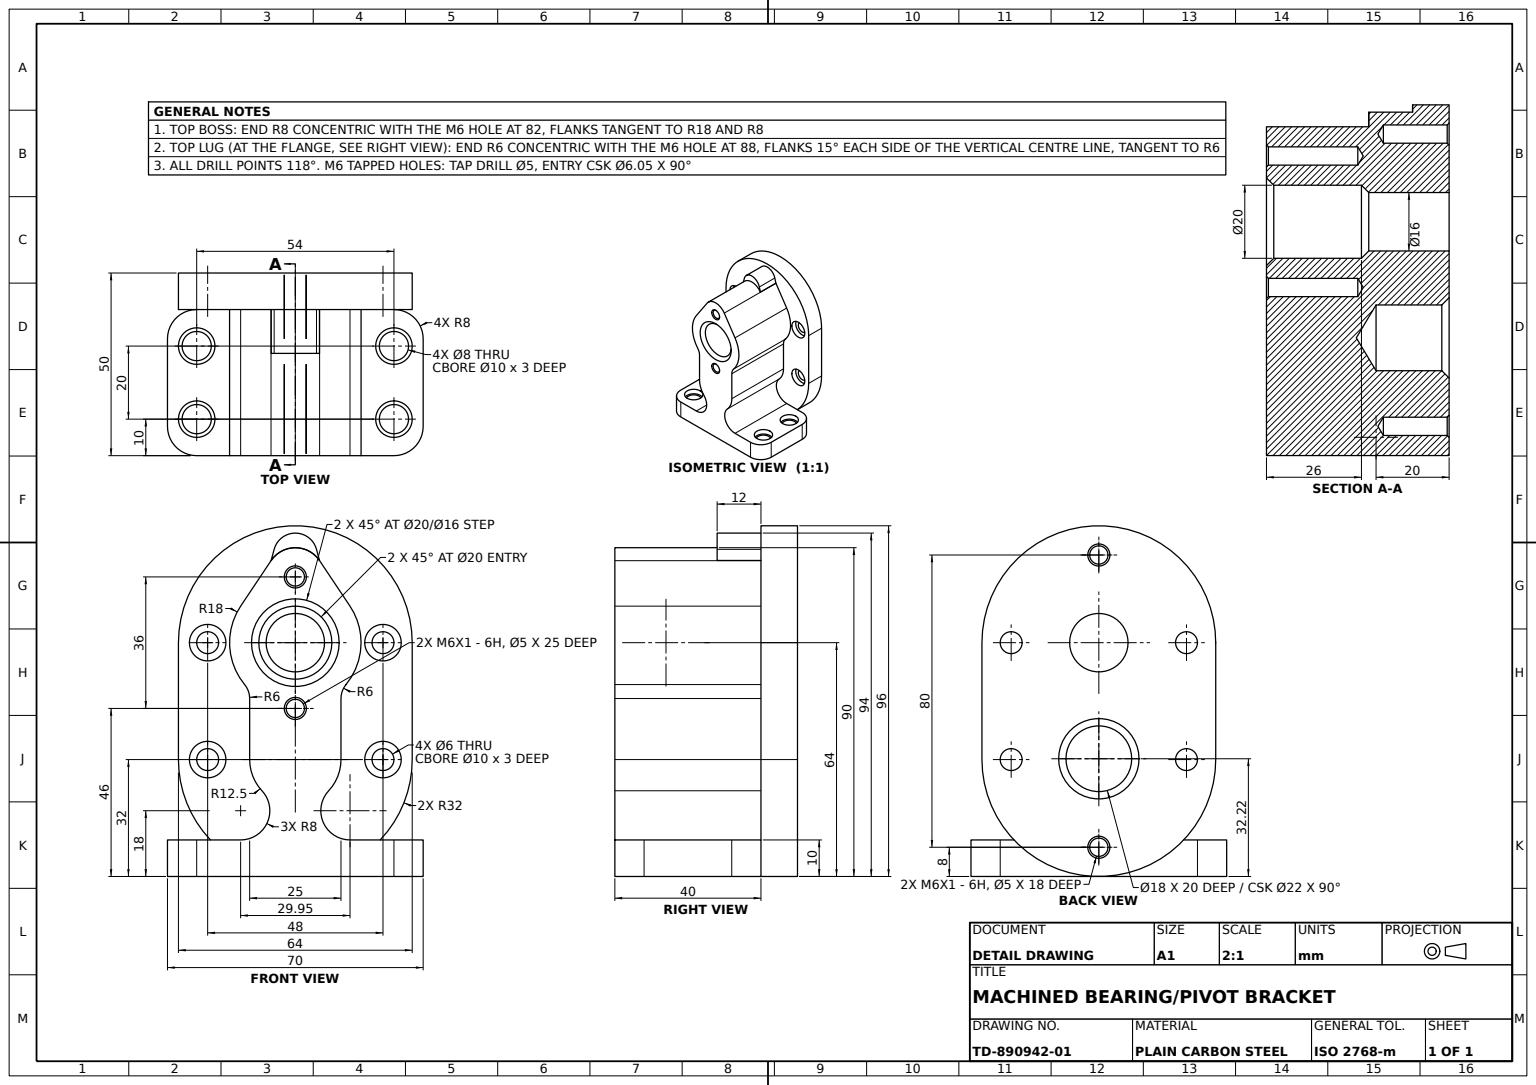
solid
v1 (19,64,-43)
v2 (29,64,-43)
e1 v1 v2 CIRCLE(AX(P(24,64,-43),D(0,0,1),D(1,0,0)),5)
v3 (19,64,-40)
e2 v1 v3 LINE
v4 (29,64,-40)
e3 v3 v4 CIRCLE(AX(P(24,64,-40),D(0,0,1),D(1,0,0)),5)
e4 v2 v4 LINE
face CYL(AX(P(24,64,-40),D(0,0,1),D(1,0,0)),5) rev [-e1 e2 e3 -e4]
v5 (2.5,82,-25)
v6 (-2.5,82,-25)
e5 v5 v6 CIRCLE(AX(P(0,82,-25),D(0,0,1),D(1,0,0)),2.5)
v7 (0,82,-26.502152)
e6 v7 v6 LINE
e7 v7 v5 LINE
face CONE(AX(P(0,82,-25),D(0,0,1),D(1,0,0)),2.5,1.029744259) rev [e5 -e6 e7]
v8 (27,32,-50)
v9 (27,32,-43)
e8 v8 v9 LINE
v10 (21,32,-43)
e9 v9 v10 CIRCLE(AX(P(24,32,-43),D(0,0,1),D(1,0,0)),3)
v11 (21,32,-50)
e10 v11 v10 LINE
e11 v8 v11 CIRCLE(AX(P(24,32,-50),D(0,0,1),D(1,0,0)),3)
face CYL(AX(P(24,32,-40),D(0,0,1),D(1,0,0)),3) rev [e8 e9 -e10 -e11]
v12 (27,7,-25)
v13 (27,7,-35)
e12 v12 v13 CIRCLE(AX(P(27,7,-30),D(0,1,0),D(0,0,1)),5)
e13 v13 v12 CIRCLE(AX(P(27,7,-30),D(0,1,0),D(0,0,1)),5)
v14 (27,7,-26)
v15 (27,7,-34)
e14 v14 v15 CIRCLE(AX(P(27,7,-30),D(0,1,0),D(0,0,1)),4)
e15 v15 v14 CIRCLE(AX(P(27,7,-30),D(0,1,0),D(0,0,1)),4)
face PLANE(AX(P(31,7,-30),D(0,-1,0),D(0,0,-1))) rev [e12 e13] [-e14 -e15]
v16 (-14.96663,74,-40)
v17 (-14.96663,74,0)
e16 v16 v17 LINE
v18 (-6.651835,86.444444,0)
e17 v18 v17 LINE
v19 (-6.651835,86.444444,-40)
e18 v19 v18 LINE
e19 v19 v16 LINE
face PLANE(AX(P(-6.651835,86.444444,-40),D(-0.831479419,0.555555556,0),D(-0.555555556,-0.831479419,0))) [e16 -e17 -e18 e19]
v20 (-21,32,-50)
v21 (-21,32,-43)
e20 v20 v21 LINE
v22 (-27,32,-50)
e21 v22 v20 CIRCLE(AX(P(-24,32,-50),D(0,0,1),D(1,0,0)),3)
v23 (-27,32,-43)
e22 v22 v23 LINE
e23 v23 v21 CIRCLE(AX(P(-24,32,-43),D(0,0,1),D(1,0,0)),3)
face CYL(AX(P(-24,32,-40),D(0,0,1),D(1,0,0)),3) rev [-e20 -e21 e22 e23]
v24 (-2.5,82,-0.525)
e24 v6 v24 LINE
v25 (2.5,82,-0.525)
e25 v24 v25 CIRCLE(AX(P(0,82,-0.525),D(0,0,1),D(1,0,0)),2.5)
e26 v5 v25 LINE
e27 v6 v5 CIRCLE(AX(P(0,82,-25),D(0,0,1),D(1,0,0)),2.5)
face CYL(AX(P(0,82,0),D(0,0,1),D(1,0,0)),2.5) rev [e24 e25 -e26 -e27]
v26 (-29,64,-43)
v27 (-19,64,-43)
e28 v26 v27 CIRCLE(AX(P(-24,64,-43),D(0,0,1),D(1,0,0)),5)
v28 (-29,64,-40)
e29 v26 v28 LINE
v29 (-19,64,-40)
e30 v28 v29 CIRCLE(AX(P(-24,64,-40),D(0,0,1),D(1,0,0)),5)
e31 v27 v29 LINE
face CYL(AX(P(-24,64,-40),D(0,0,1),D(1,0,0)),5) rev [-e28 e29 e30 -e31]
v30 (8,64,-28)
v31 (10,64,-26)
e32 v30 v31 LINE
v32 (-10,64,-26)
e33 v32 v31 CIRCLE(AX(P(0,64,-26),D(0,0,-1),D(1,0,0)),10)
v33 (-8,64,-28)
e34 v33 v32 LINE
e35 v30 v33 CIRCLE(AX(P(0,64,-28),D(0,0,1),D(1,0,0)),8)
face CONE(AX(P(0,64,-28),D(0,0,1),D(1,0,0)),8,0.785398163) rev [e32 -e33 -e34 -e35]
v34 (27,64,-43)
v35 (21,64,-43)
e36 v34 v35 CIRCLE(AX(P(24,64,-43),D(0,0,1),D(1,0,0)),3)
v36 (21,64,-50)
e37 v36 v35 LINE
v37 (27,64,-50)
e38 v37 v36 CIRCLE(AX(P(24,64,-50),D(0,0,1),D(1,0,0)),3)
e39 v37 v34 LINE
face CYL(AX(P(24,64,-40),D(0,0,1),D(1,0,0)),3) rev [e36 -e37 -e38 e39]
v38 (2.5,46,-25)
v39 (-2.5,46,-25)
e40 v38 v39 CIRCLE(AX(P(0,46,-25),D(0,0,1),D(1,0,0)),2.5)
v40 (2.5,46,-0.525)
e41 v38 v40 LINE
v41 (-2.5,46,-0.525)
e42 v40 v41 CIRCLE(AX(P(0,46,-0.525),D(0,0,1),D(1,0,0)),2.5)
e43 v39 v41 LINE
face CYL(AX(P(0,46,0),D(0,0,1),D(1,0,0)),2.5) rev [-e40 e41 e42 -e43]
e44 v41 v40 CIRCLE(AX(P(0,46,-0.525),D(0,0,1),D(1,0,0)),2.5)
e45 v39 v38 CIRCLE(AX(P(0,46,-25),D(0,0,1),D(1,0,0)),2.5)
face CYL(AX(P(0,46,0),D(0,0,1),D(1,0,0)),2.5) rev [e43 e44 -e41 -e45]
v42 (27,7,-14)
v43 (27,7,-6)
e46 v42 v43 CIRCLE(AX(P(27,7,-10),D(0,1,0),D(0,0,1)),4)
v44 (27,0,-6)
e47 v44 v43 LINE
v45 (27,0,-14)
e48 v45 v44 CIRCLE(AX(P(27,0,-10),D(0,1,0),D(0,0,1)),4)
e49 v45 v42 LINE
face CYL(AX(P(27,10,-10),D(0,1,0),D(0,0,1)),4) rev [e46 -e47 -e48 e49]
v46 (0,8,-30.497848)
v47 (2.5,8,-32)
e50 v46 v47 LINE
v48 (-2.5,8,-32)
e51 v46 v48 LINE
e52 v48 v47 CIRCLE(AX(P(0,8,-32),D(0,0,-1),D(-1,0,0)),2.5)
face CONE(AX(P(0,8,-32),D(0,0,-1),D(-1,0,0)),2.5,1.029744259) rev [-e50 e51 e52]
v49 (-27,7,-15)
v50 (-27,10,-15)
e53 v49 v50 LINE
v51 (-27,7,-5)
e54 v51 v49 CIRCLE(AX(P(-27,7,-10),D(0,1,0),D(0,0,1)),5)
v52 (-27,10,-5)
e55 v51 v52 LINE
e56 v52 v50 CIRCLE(AX(P(-27,10,-10),D(0,1,0),D(0,0,1)),5)
face CYL(AX(P(-27,10,-10),D(0,1,0),D(0,0,1)),5) rev [-e53 -e54 e55 e56]
v53 (-27,7,-35)
v54 (-27,10,-35)
e57 v53 v54 LINE
v55 (-27,10,-25)
e58 v54 v55 CIRCLE(AX(P(-27,10,-30),D(0,1,0),D(0,0,1)),5)
v56 (-27,7,-25)
e59 v56 v55 LINE
e60 v53 v56 CIRCLE(AX(P(-27,7,-30),D(0,1,0),D(0,0,1)),5)
face CYL(AX(P(-27,10,-30),D(0,1,0),D(0,0,1)),5) rev [e57 e58 -e59 -e60]
v57 (32,64,-50)
v58 (32,32,-50)
e61 v57 v58 LINE
v59 (32,64,-40)
e62 v57 v59 LINE
v60 (32,32,-40)
e63 v59 v60 LINE
e64 v58 v60 LINE
face PLANE(AX(P(32,64,-50),D(-1,0,0),D(0,0,1))) rev [-e61 e62 e63 -e64]
v61 (-12.5,32,0)
v62 (-9.131085,23.463415,0)
e65 v61 v62 CIRCLE(AX(P(0,32,0),D(0,0,1),D(-1,0,0)),12.5)
v63 (-12.5,32,-40)
e66 v63 v61 LINE
v64 (-9.131085,23.463415,-40)
e67 v63 v64 CIRCLE(AX(P(0,32,-40),D(0,0,1),D(-1,0,0)),12.5)
e68 v64 v62 LINE
face CYL(AX(P(0,32,-40),D(0,0,1),D(1,0,0)),12.5) [-e65 -e66 e67 e68]
v65 (-5.795555,89.552914,-28)
v66 (-5.795555,89.552914,-40)
e69 v65 v66 LINE
v67 (5.795555,89.552914,-28)
e70 v67 v65 CIRCLE(AX(P(0,88,-28),D(0,0,1),D(1,0,0)),6)
v68 (5.795555,89.552914,-40)
e71 v67 v68 LINE
e72 v68 v66 CIRCLE(AX(P(0,88,-40),D(0,0,1),D(1,0,0)),6)
face CYL(AX(P(0,88,-28),D(0,0,-1),D(-1,0,0)),6) [-e69 -e70 e71 e72]
v69 (-21,64,-43)
v70 (-27,64,-43)
e73 v69 v70 CIRCLE(AX(P(-24,64,-43),D(0,0,1),D(1,0,0)),3)
e74 v70 v69 CIRCLE(AX(P(-24,64,-43),D(0,0,1),D(1,0,0)),3)
e75 v27 v26 CIRCLE(AX(P(-24,64,-43),D(0,0,1),D(1,0,0)),5)
face PLANE(AX(P(-21,64,-43),D(0,0,-1),D(-1,0,0))) rev [-e73 -e74] [e28 e75]
e76 v50 v52 CIRCLE(AX(P(-27,10,-10),D(0,1,0),D(0,0,1)),5)
e77 v49 v51 CIRCLE(AX(P(-27,7,-10),D(0,1,0),D(0,0,1)),5)
face CYL(AX(P(-27,10,-10),D(0,1,0),D(0,0,1)),5) rev [e76 -e55 -e77 e53]
v71 (9.131085,23.463415,-40)
v72 (9.131085,23.463415,0)
e78 v71 v72 LINE
v73 (12.5,32,-40)
e79 v71 v73 CIRCLE(AX(P(0,32,-40),D(0,0,1),D(1,0,0)),12.5)
v74 (12.5,32,0)
e80 v73 v74 LINE
e81 v72 v74 CIRCLE(AX(P(0,32,0),D(0,0,1),D(1,0,0)),12.5)
face CYL(AX(P(0,32,-40),D(0,0,1),D(1,0,0)),12.5) [-e78 e79 e80 -e81]
e82 v55 v54 CIRCLE(AX(P(-27,10,-30),D(0,1,0),D(0,0,1)),5)
e83 v56 v53 CIRCLE(AX(P(-27,7,-30),D(0,1,0),D(0,0,1)),5)
face CYL(AX(P(-27,10,-30),D(0,1,0),D(0,0,1)),5) rev [e82 -e57 -e83 e59]
v75 (10,64,-2)
v76 (-10,64,-2)
e84 v75 v76 CIRCLE(AX(P(0,64,-2),D(0,0,1),D(-1,0,0)),10)
v77 (12,64,0)
e85 v75 v77 LINE
v78 (-12,64,0)
e86 v78 v77 CIRCLE(AX(P(0,64,0),D(0,0,-1),D(-1,0,0)),12)
e87 v76 v78 LINE
face CONE(AX(P(0,64,-2),D(0,0,1),D(1,0,0)),10,0.785398163) rev [-e84 e85 -e86 -e87]
v79 (-27,7,-34)
v80 (-27,7,-26)
e88 v79 v80 CIRCLE(AX(P(-27,7,-30),D(0,1,0),D(0,0,1)),4)
e89 v80 v79 CIRCLE(AX(P(-27,7,-30),D(0,1,0),D(0,0,1)),4)
face PLANE(AX(P(-23,7,-30),D(0,-1,0),D(0,0,-1))) rev [-e88 -e89] [e83 e60]
v81 (-8,64,-50)
e90 v81 v33 LINE
v82 (8,64,-50)
e91 v82 v81 CIRCLE(AX(P(0,64,-50),D(0,0,1),D(1,0,0)),8)
e92 v82 v30 LINE
face CYL(AX(P(0,64,15.77033),D(0,0,1),D(1,0,0)),8) rev [-e90 -e91 e92 e35]
v83 (35,10,-32)
v84 (35,10,-8)
e93 v83 v84 LINE
v85 (35,0,-8)
e94 v84 v85 LINE
v86 (35,0,-32)
e95 v86 v85 LINE
e96 v86 v83 LINE
face PLANE(AX(P(35,0,-40),D(1,0,0),D(0,1,0))) [e93 e94 -e95 e96]
v87 (0,0,-40)
v88 (-23.2379,10,-40)
e97 v87 v88 CIRCLE(AX(P(0,32,-40),D(0,0,-1),D(-1,0,0)),32)
v89 (-32,32,-40)
e98 v88 v89 CIRCLE(AX(P(0,32,-40),D(0,0,-1),D(-1,0,0)),32)
v90 (-32,32,-50)
e99 v90 v89 LINE
e100 v58 v90 CIRCLE(AX(P(0,32,-50),D(0,0,-1),D(-1,0,0)),32)
v91 (23.2379,10,-40)
e101 v60 v91 CIRCLE(AX(P(0,32,-40),D(0,0,-1),D(-1,0,0)),32)
e102 v91 v87 CIRCLE(AX(P(0,32,-40),D(0,0,-1),D(-1,0,0)),32)
face CYL(AX(P(0,32,-50),D(0,0,1),D(1,0,0)),32) [e97 e98 -e99 -e100 e64 e101 e102]
e103 v2 v1 CIRCLE(AX(P(24,64,-43),D(0,0,1),D(1,0,0)),5)
e104 v4 v3 CIRCLE(AX(P(24,64,-40),D(0,0,1),D(1,0,0)),5)
face CYL(AX(P(24,64,-40),D(0,0,1),D(1,0,0)),5) rev [-e103 e4 e104 -e2]
v92 (2.5,8,-49.475)
v93 (-2.5,8,-49.475)
e105 v92 v93 CIRCLE(AX(P(0,8,-49.475),D(0,0,-1),D(-1,0,0)),2.5)
e106 v48 v93 LINE
e107 v47 v48 CIRCLE(AX(P(0,8,-32),D(0,0,-1),D(-1,0,0)),2.5)
e108 v47 v92 LINE
face CYL(AX(P(0,8,-50),D(0,0,-1),D(-1,0,0)),2.5) rev [e105 -e106 -e107 e108]
v94 (27,7,-5)
v95 (27,10,-5)
e109 v94 v95 LINE
v96 (27,7,-15)
e110 v96 v94 CIRCLE(AX(P(27,7,-10),D(0,1,0),D(0,0,1)),5)
v97 (27,10,-15)
e111 v96 v97 LINE
e112 v97 v95 CIRCLE(AX(P(27,10,-10),D(0,1,0),D(0,0,1)),5)
face CYL(AX(P(27,10,-10),D(0,1,0),D(0,0,1)),5) rev [-e109 -e110 e111 e112]
v98 (-3.025,8,-50)
v99 (3.025,8,-50)
e113 v98 v99 CIRCLE(AX(P(0,8,-50),D(0,0,-1),D(-1,0,0)),3.025)
e114 v92 v99 LINE
e115 v93 v92 CIRCLE(AX(P(0,8,-49.475),D(0,0,-1),D(-1,0,0)),2.5)
e116 v93 v98 LINE
face CONE(AX(P(0,8,-50),D(0,0,-1),D(-1,0,0)),3.025,0.785398163) rev [e113 -e114 -e115 e116]
v100 (-6.613063,86.501933,-28)
e117 v65 v100 LINE
v101 (6.613063,86.501933,-28)
e118 v100 v101 CIRCLE(AX(P(0,82,-28),D(0,0,-1),D(1,0,0)),8)
e119 v101 v67 LINE
face PLANE(AX(P(0,88,-28),D(0,0,1),D(1,0,0))) [e117 e118 e119 e70]
v102 (27,0,-40)
e120 v102 v86 CIRCLE(AX(P(27,0,-32),D(0,-1,0),D(0,0,-1)),8)
v103 (27,10,-40)
e121 v103 v102 LINE
e122 v83 v103 CIRCLE(AX(P(27,10,-32),D(0,1,0),D(-1,0,0)),8)
face CYL(AX(P(27,0,-32),D(0,1,0),D(-1,0,0)),8) [-e96 -e120 -e121 -e122]
v104 (-6.974979,18,-40)
v105 (-14.974979,10,-40)
e123 v104 v105 CIRCLE(AX(P(-14.974979,18,-40),D(0,0,-1),D(1,0,0)),8)
v106 (-14.974979,10,0)
e124 v105 v106 LINE
v107 (-6.974979,18,0)
e125 v107 v106 CIRCLE(AX(P(-14.974979,18,0),D(0,0,-1),D(1,0,0)),8)
e126 v104 v107 LINE
face CYL(AX(P(-14.974979,18,-40),D(0,0,1),D(1,0,0)),8) rev [e123 e124 -e125 -e126]
face CYL(AX(P(0,8,-50),D(0,0,-1),D(-1,0,0)),2.5) rev [e106 e115 -e108 -e52]
e127 v10 v9 CIRCLE(AX(P(24,32,-43),D(0,0,1),D(1,0,0)),3)
e128 v11 v8 CIRCLE(AX(P(24,32,-50),D(0,0,1),D(1,0,0)),3)
face CYL(AX(P(24,32,-40),D(0,0,1),D(1,0,0)),3) rev [e10 e127 -e8 -e128]
v108 (-29,32,-43)
v109 (-19,32,-43)
e129 v108 v109 CIRCLE(AX(P(-24,32,-43),D(0,0,1),D(1,0,0)),5)
e130 v109 v108 CIRCLE(AX(P(-24,32,-43),D(0,0,1),D(1,0,0)),5)
e131 v21 v23 CIRCLE(AX(P(-24,32,-43),D(0,0,1),D(1,0,0)),3)
face PLANE(AX(P(-21,32,-43),D(0,0,-1),D(-1,0,0))) rev [e129 e130] [-e23 -e131]
v110 (27,10,-25)
v111 (27,10,-35)
e132 v110 v111 CIRCLE(AX(P(27,10,-30),D(0,1,0),D(0,0,1)),5)
e133 v111 v110 CIRCLE(AX(P(27,10,-30),D(0,1,0),D(0,0,1)),5)
v112 (27,10,0)
e134 v112 v84 CIRCLE(AX(P(27,10,-8),D(0,1,0),D(-1,0,0)),8)
e135 v103 v91 LINE
v113 (14.974979,10,-40)
e136 v91 v113 LINE
v114 (14.974979,10,0)
e137 v113 v114 LINE
e138 v112 v114 LINE
e139 v95 v97 CIRCLE(AX(P(27,10,-10),D(0,1,0),D(0,0,1)),5)
face PLANE(AX(P(35,10,-40),D(0,1,0),D(-1,0,0))) [-e132 -e133] [e134 -e93 e122 e135 e136 e137 -e138] [-e112 -e139]
v115 (3.025,46,0)
e140 v40 v115 LINE
v116 (-3.025,46,0)
e141 v41 v116 LINE
e142 v116 v115 CIRCLE(AX(P(0,46,0),D(0,0,1),D(1,0,0)),3.025)
face CONE(AX(P(0,46,0),D(0,0,1),D(1,0,0)),3.025,0.785398163) rev [-e140 -e44 e141 e142]
v117 (-21,64,-50)
v118 (-27,64,-50)
e143 v117 v118 CIRCLE(AX(P(-24,64,-50),D(0,0,1),D(1,0,0)),3)
e144 v117 v69 LINE
e145 v118 v70 LINE
face CYL(AX(P(-24,64,-40),D(0,0,1),D(1,0,0)),3) rev [-e143 e144 e73 -e145]
e146 v115 v116 CIRCLE(AX(P(0,46,0),D(0,0,1),D(1,0,0)),3.025)
face CONE(AX(P(0,46,0),D(0,0,1),D(1,0,0)),3.025,0.785398163) rev [-e42 e140 e146 -e141]
e147 v25 v24 CIRCLE(AX(P(0,82,-0.525),D(0,0,1),D(1,0,0)),2.5)
face CYL(AX(P(0,82,0),D(0,0,1),D(1,0,0)),2.5) rev [e26 e147 -e24 -e5]
v119 (2.5,88,-32)
v120 (2.5,88,-49.475)
e148 v119 v120 LINE
v121 (-2.5,88,-32)
e149 v121 v119 CIRCLE(AX(P(0,88,-32),D(0,0,-1),D(-1,0,0)),2.5)
v122 (-2.5,88,-49.475)
e150 v121 v122 LINE
e151 v122 v120 CIRCLE(AX(P(0,88,-49.475),D(0,0,-1),D(-1,0,0)),2.5)
face CYL(AX(P(0,88,-50),D(0,0,-1),D(-1,0,0)),2.5) rev [-e148 -e149 e150 e151]
v123 (3.025,82,0)
e152 v25 v123 LINE
v124 (-3.025,82,0)
e153 v123 v124 CIRCLE(AX(P(0,82,0),D(0,0,1),D(1,0,0)),3.025)
e154 v24 v124 LINE
face CONE(AX(P(0,82,0),D(0,0,1),D(1,0,0)),3.025,0.785398163) rev [e152 e153 -e154 -e147]
e155 v31 v75 LINE
e156 v32 v76 LINE
face CYL(AX(P(0,64,15.77033),D(0,0,1),D(1,0,0)),10) rev [e155 e84 -e156 e33]
v125 (27,0,-26)
e157 v125 v14 LINE
v126 (27,0,-34)
e158 v126 v125 CIRCLE(AX(P(27,0,-30),D(0,1,0),D(0,0,1)),4)
e159 v126 v15 LINE
face CYL(AX(P(27,10,-30),D(0,1,0),D(0,0,1)),4) rev [e15 -e157 -e158 e159]
v127 (14.96663,74,-40)
v128 (14.96663,74,0)
e160 v127 v128 LINE
v129 (18,64,0)
e161 v129 v128 CIRCLE(AX(P(0,64,0),D(0,0,1),D(1,0,0)),18)
v130 (18,64,-40)
e162 v130 v129 LINE
e163 v130 v127 CIRCLE(AX(P(0,64,-40),D(0,0,1),D(1,0,0)),18)
face CYL(AX(P(0,64,-40),D(0,0,1),D(1,0,0)),18) [e160 -e161 -e162 e163]
e164 v29 v28 CIRCLE(AX(P(-24,64,-40),D(0,0,1),D(1,0,0)),5)
face CYL(AX(P(-24,64,-40),D(0,0,1),D(1,0,0)),5) rev [e164 -e29 -e75 e31]
v131 (6.651835,86.444444,-40)
v132 (6.651835,86.444444,0)
e165 v131 v132 LINE
v133 (6.613063,86.501933,-40)
e166 v131 v133 CIRCLE(AX(P(0,82,-40),D(0,0,1),D(1,0,0)),8)
e167 v101 v133 LINE
v134 (-6.613063,86.501933,-40)
e168 v100 v134 LINE
e169 v134 v19 CIRCLE(AX(P(0,82,-40),D(0,0,1),D(1,0,0)),8)
e170 v132 v18 CIRCLE(AX(P(0,82,0),D(0,0,1),D(1,0,0)),8)
face CYL(AX(P(0,82,-40),D(0,0,1),D(1,0,0)),8) [-e165 e166 -e167 -e118 e168 e169 e18 -e170]
e171 v12 v110 LINE
e172 v13 v111 LINE
face CYL(AX(P(27,10,-30),D(0,1,0),D(0,0,1)),5) rev [e133 -e171 -e13 e172]
face CONE(AX(P(0,82,-25),D(0,0,1),D(1,0,0)),2.5,1.029744259) rev [-e7 e6 e27]
v135 (-13.875,52.533336,-40)
e173 v16 v135 CIRCLE(AX(P(0,64,-40),D(0,0,1),D(1,0,0)),18)
v136 (-13.875,52.533336,0)
e174 v135 v136 LINE
e175 v17 v136 CIRCLE(AX(P(0,64,0),D(0,0,1),D(1,0,0)),18)
face CYL(AX(P(0,64,-40),D(0,0,1),D(1,0,0)),18) [-e16 e173 e174 -e175]
v137 (9,32.224907,-30)
v138 (9,32.224907,-48)
e176 v137 v138 LINE
v139 (-9,32.224907,-48)
e177 v138 v139 CIRCLE(AX(P(0,32.224907,-48),D(0,0,-1),D(-1,0,0)),9)
v140 (-9,32.224907,-30)
e178 v140 v139 LINE
e179 v137 v140 CIRCLE(AX(P(0,32.224907,-30),D(0,0,-1),D(-1,0,0)),9)
face CYL(AX(P(0,32.224907,-50),D(0,0,-1),D(-1,0,0)),9) rev [e176 e177 -e178 -e179]
v141 (0,32.224907,-24.592254)
e180 v141 v140 LINE
e181 v141 v137 LINE
face CONE(AX(P(0,32.224907,-30),D(0,0,-1),D(-1,0,0)),9,1.029744259) rev [e179 -e180 e181]
e182 v118 v117 CIRCLE(AX(P(-24,64,-50),D(0,0,1),D(1,0,0)),3)
face CYL(AX(P(-24,64,-40),D(0,0,1),D(1,0,0)),3) rev [e74 -e144 -e182 e145]
face CYL(AX(P(27,10,-30),D(0,1,0),D(0,0,1)),5) rev [-e172 -e12 e171 e132]
v142 (-27,0,-6)
v143 (-27,0,-14)
e183 v142 v143 CIRCLE(AX(P(-27,0,-10),D(0,1,0),D(0,0,1)),4)
e184 v143 v142 CIRCLE(AX(P(-27,0,-10),D(0,1,0),D(0,0,1)),4)
e185 v44 v45 CIRCLE(AX(P(27,0,-10),D(0,1,0),D(0,0,1)),4)
v144 (-27,0,-34)
v145 (-27,0,-26)
e186 v144 v145 CIRCLE(AX(P(-27,0,-30),D(0,1,0),D(0,0,1)),4)
e187 v145 v144 CIRCLE(AX(P(-27,0,-30),D(0,1,0),D(0,0,1)),4)
e188 v125 v126 CIRCLE(AX(P(27,0,-30),D(0,1,0),D(0,0,1)),4)
v146 (27,0,0)
e189 v85 v146 CIRCLE(AX(P(27,0,-8),D(0,-1,0),D(0,0,-1)),8)
v147 (-27,0,0)
e190 v147 v146 LINE
v148 (-35,0,-8)
e191 v147 v148 CIRCLE(AX(P(-27,0,-8),D(0,-1,0),D(0,0,-1)),8)
v149 (-35,0,-32)
e192 v149 v148 LINE
v150 (-27,0,-40)
e193 v149 v150 CIRCLE(AX(P(-27,0,-32),D(0,-1,0),D(0,0,-1)),8)
e194 v150 v87 LINE
e195 v87 v102 LINE
face PLANE(AX(P(-35,0,-40),D(0,-1,0),D(0,0,-1))) [e183 e184] [e48 e185] [e186 e187] [e158 e188] [e189 -e190 e191 -e192 e193 e194 e195 e120 e95]
e196 v133 v68 LINE
face PLANE(AX(P(5.795555,89.552914,-28),D(-0.965925826,-0.258819045,0),D(0.258819045,-0.965925826,0))) rev [-e119 e167 e196 -e71]
e197 v43 v42 CIRCLE(AX(P(27,7,-10),D(0,1,0),D(0,0,1)),4)
face CYL(AX(P(27,10,-10),D(0,1,0),D(0,0,1)),4) rev [e197 -e49 -e185 e47]
face CYL(AX(P(27,10,-30),D(0,1,0),D(0,0,1)),4) rev [e14 -e159 -e188 e157]
e198 v124 v123 CIRCLE(AX(P(0,82,0),D(0,0,1),D(1,0,0)),3.025)
e199 v77 v78 CIRCLE(AX(P(0,64,0),D(0,0,-1),D(-1,0,0)),12)
e200 v128 v132 LINE
v151 (-12.5,48.711115,0)
e201 v136 v151 CIRCLE(AX(P(-18.5,48.711115,0),D(0,0,-1),D(1,0,0)),6)
e202 v151 v61 LINE
e203 v62 v107 CIRCLE(AX(P(-14.974979,18,0),D(0,0,-1),D(1,0,0)),8)
v152 (-27,10,0)
e204 v106 v152 LINE
e205 v152 v147 LINE
e206 v146 v112 LINE
e207 v114 v72 CIRCLE(AX(P(14.974979,18,0),D(0,0,-1),D(-1,0,0)),8)
v153 (12.5,48.711115,0)
e208 v74 v153 LINE
v154 (13.875,52.533336,0)
e209 v153 v154 CIRCLE(AX(P(18.5,48.711115,0),D(0,0,-1),D(-1,0,0)),6)
e210 v154 v129 CIRCLE(AX(P(0,64,0),D(0,0,1),D(1,0,0)),18)
face PLANE(AX(P(14.974979,18,0),D(0,0,-1),D(-1,0,0))) rev [-e198 -e153] [e86 e199] [-e146 -e142] [e161 e200 e170 e17 e175 e201 e202 e65 e203 e125 e204 e205 e190 e206 e138 e207 e81 e208 e209 e210]
v155 (19,32,-40)
v156 (29,32,-40)
e211 v155 v156 CIRCLE(AX(P(24,32,-40),D(0,0,1),D(1,0,0)),5)
e212 v156 v155 CIRCLE(AX(P(24,32,-40),D(0,0,1),D(1,0,0)),5)
v157 (-29,32,-40)
v158 (-19,32,-40)
e213 v157 v158 CIRCLE(AX(P(-24,32,-40),D(0,0,1),D(1,0,0)),5)
e214 v158 v157 CIRCLE(AX(P(-24,32,-40),D(0,0,1),D(1,0,0)),5)
e215 v127 v131 LINE
v159 (13.875,52.533336,-40)
e216 v159 v130 CIRCLE(AX(P(0,64,-40),D(0,0,1),D(1,0,0)),18)
v160 (12.5,48.711115,-40)
e217 v160 v159 CIRCLE(AX(P(18.5,48.711115,-40),D(0,0,-1),D(-1,0,0)),6)
e218 v73 v160 LINE
e219 v113 v71 CIRCLE(AX(P(14.974979,18,-40),D(0,0,-1),D(-1,0,0)),8)
v161 (-32,64,-40)
e220 v161 v59 CIRCLE(AX(P(0,64,-40),D(0,0,-1),D(-1,0,0)),32)
e221 v89 v161 LINE
e222 v105 v88 LINE
e223 v64 v104 CIRCLE(AX(P(-14.974979,18,-40),D(0,0,-1),D(1,0,0)),8)
v162 (-12.5,48.711115,-40)
e224 v162 v63 LINE
e225 v135 v162 CIRCLE(AX(P(-18.5,48.711115,-40),D(0,0,-1),D(1,0,0)),6)
e226 v66 v134 LINE
face PLANE(AX(P(0,64,-40),D(0,0,-1),D(-1,0,0))) rev [-e211 -e212] [-e164 -e30] [-e213 -e214] [-e215 -e163 -e216 -e217 -e218 -e79 -e219 -e136 -e101 -e63 -e220 -e221 -e98 -e222 -e123 -e223 -e67 -e224 -e225 -e173 -e19 -e169 -e226 -e72 -e196 -e166] [-e104 -e3]
v163 (-27,7,-14)
e227 v143 v163 LINE
v164 (-27,7,-6)
e228 v163 v164 CIRCLE(AX(P(-27,7,-10),D(0,1,0),D(0,0,1)),4)
e229 v142 v164 LINE
face CYL(AX(P(-27,10,-10),D(0,1,0),D(0,0,1)),4) rev [e227 e228 -e229 -e184]
e230 v140 v137 CIRCLE(AX(P(0,32.224907,-30),D(0,0,-1),D(-1,0,0)),9)
e231 v139 v138 CIRCLE(AX(P(0,32.224907,-48),D(0,0,-1),D(-1,0,0)),9)
face CYL(AX(P(0,32.224907,-50),D(0,0,-1),D(-1,0,0)),9) rev [-e176 -e230 e178 e231]
face CONE(AX(P(0,82,0),D(0,0,1),D(1,0,0)),3.025,0.785398163) rev [-e152 -e25 e154 e198]
face PLANE(AX(P(6.651835,86.444444,-40),D(0.831479419,0.555555556,0),D(-0.555555556,0.831479419,0))) [e165 -e200 -e160 e215]
e232 v35 v34 CIRCLE(AX(P(24,64,-43),D(0,0,1),D(1,0,0)),3)
face PLANE(AX(P(27,64,-43),D(0,0,-1),D(-1,0,0))) rev [e1 e103] [-e36 -e232]
v165 (0,46,-26.502152)
e233 v165 v38 LINE
e234 v165 v39 LINE
face CONE(AX(P(0,46,-25),D(0,0,1),D(1,0,0)),2.5,1.029744259) rev [e45 -e233 e234]
e235 v159 v154 LINE
face CYL(AX(P(0,64,-40),D(0,0,1),D(1,0,0)),18) [e216 e162 -e210 -e235]
v166 (3.025,88,-50)
e236 v120 v166 LINE
v167 (-3.025,88,-50)
e237 v122 v167 LINE
e238 v167 v166 CIRCLE(AX(P(0,88,-50),D(0,0,-1),D(-1,0,0)),3.025)
face CONE(AX(P(0,88,-50),D(0,0,-1),D(-1,0,0)),3.025,0.785398163) rev [-e236 -e151 e237 e238]
v168 (-35,10,-8)
e239 v168 v152 CIRCLE(AX(P(-27,10,-8),D(0,1,0),D(-1,0,0)),8)
e240 v148 v168 LINE
face CYL(AX(P(-27,18,-8),D(0,1,0),D(-1,0,0)),8) [-e205 -e239 -e240 -e191]
e241 v120 v122 CIRCLE(AX(P(0,88,-49.475),D(0,0,-1),D(-1,0,0)),2.5)
e242 v119 v121 CIRCLE(AX(P(0,88,-32),D(0,0,-1),D(-1,0,0)),2.5)
face CYL(AX(P(0,88,-50),D(0,0,-1),D(-1,0,0)),2.5) rev [e148 e241 -e150 -e242]
e243 v166 v167 CIRCLE(AX(P(0,88,-50),D(0,0,-1),D(-1,0,0)),3.025)
face CONE(AX(P(0,88,-50),D(0,0,-1),D(-1,0,0)),3.025,0.785398163) rev [-e241 e236 e243 -e237]
e244 v76 v75 CIRCLE(AX(P(0,64,-2),D(0,0,1),D(-1,0,0)),10)
face CONE(AX(P(0,64,-2),D(0,0,1),D(1,0,0)),10,0.785398163) rev [-e244 e87 -e199 -e85]
e245 v99 v98 CIRCLE(AX(P(0,8,-50),D(0,0,-1),D(-1,0,0)),3.025)
face CONE(AX(P(0,8,-50),D(0,0,-1),D(-1,0,0)),3.025,0.785398163) rev [-e116 -e105 e114 e245]
e246 v109 v158 LINE
e247 v108 v157 LINE
face CYL(AX(P(-24,32,-40),D(0,0,1),D(1,0,0)),5) rev [-e130 e246 e214 -e247]
v169 (-32,64,-50)
e248 v169 v57 CIRCLE(AX(P(0,64,-50),D(0,0,-1),D(-1,0,0)),32)
e249 v169 v161 LINE
face CYL(AX(P(0,64,-50),D(0,0,1),D(1,0,0)),32) [-e248 e249 e220 -e62]
e250 v81 v82 CIRCLE(AX(P(0,64,-50),D(0,0,1),D(1,0,0)),8)
e251 v36 v37 CIRCLE(AX(P(24,64,-50),D(0,0,1),D(1,0,0)),3)
v170 (-11,32.224907,-50)
v171 (11,32.224907,-50)
e252 v170 v171 CIRCLE(AX(P(0,32.224907,-50),D(0,0,1),D(-1,0,0)),11)
e253 v171 v170 CIRCLE(AX(P(0,32.224907,-50),D(0,0,1),D(-1,0,0)),11)
e254 v90 v169 LINE
e255 v20 v22 CIRCLE(AX(P(-24,32,-50),D(0,0,1),D(1,0,0)),3)
face PLANE(AX(P(0,64,-50),D(0,0,-1),D(-1,0,0))) [e250 e91] [e251 e38] [e252 e253] [e182 e143] [-e243 -e238] [e248 e61 e100 e254] [-e113 -e245] [e11 e128] [e255 e21]
v172 (-27,10,-40)
v173 (-35,10,-32)
e256 v172 v173 CIRCLE(AX(P(-27,10,-32),D(0,1,0),D(-1,0,0)),8)
e257 v150 v172 LINE
e258 v173 v149 LINE
face CYL(AX(P(-27,0,-32),D(0,-1,0),D(1,0,0)),8) [-e256 -e257 -e193 -e258]
face PLANE(AX(P(-5.795555,89.552914,-28),D(0.965925826,-0.258819045,0),D(0.258819045,0.965925826,0))) rev [e69 e226 -e168 -e117]
face CYL(AX(P(14.974979,18,-40),D(0,0,1),D(1,0,0)),8) rev [-e137 e219 e78 -e207]
e259 v33 v30 CIRCLE(AX(P(0,64,-28),D(0,0,1),D(1,0,0)),8)
face CYL(AX(P(0,64,15.77033),D(0,0,1),D(1,0,0)),8) rev [-e250 e90 e259 -e92]
face PLANE(AX(P(-32,64,-50),D(1,0,0),D(0,1,0))) rev [-e254 e99 e221 -e249]
face CYL(AX(P(-24,32,-40),D(0,0,1),D(1,0,0)),3) rev [e131 -e22 -e255 e20]
face CONE(AX(P(0,32.224907,-30),D(0,0,-1),D(-1,0,0)),9,1.029744259) rev [e230 -e181 e180]
face PLANE(AX(P(14.974979,18,-40),D(0,0,-1),D(-1,0,0))) [e121 -e195 -e102 -e135]
e260 v164 v163 CIRCLE(AX(P(-27,7,-10),D(0,1,0),D(0,0,1)),4)
face CYL(AX(P(-27,10,-10),D(0,1,0),D(0,0,1)),4) rev [-e227 -e183 e229 e260]
v174 (0,88,-30.497848)
e261 v174 v121 LINE
e262 v174 v119 LINE
face CONE(AX(P(0,88,-32),D(0,0,-1),D(-1,0,0)),2.5,1.029744259) rev [-e261 e262 e242]
e263 v173 v168 LINE
face PLANE(AX(P(-35,0,-40),D(-1,0,0),D(0,-1,0))) [e192 e240 -e263 e258]
e264 v138 v171 LINE
e265 v139 v170 LINE
face CONE(AX(P(0,32.224907,-48),D(0,0,-1),D(-1,0,0)),9,0.785398163) rev [-e264 -e231 e265 -e253]
face CYL(AX(P(24,64,-40),D(0,0,1),D(1,0,0)),3) rev [e232 -e39 -e251 e37]
e266 v94 v96 CIRCLE(AX(P(27,7,-10),D(0,1,0),D(0,0,1)),5)
face CYL(AX(P(27,10,-10),D(0,1,0),D(0,0,1)),5) rev [e109 e139 -e111 -e266]
face CONE(AX(P(0,32.224907,-48),D(0,0,-1),D(-1,0,0)),9,0.785398163) rev [-e177 e264 -e252 -e265]
face CONE(AX(P(0,8,-32),D(0,0,-1),D(-1,0,0)),2.5,1.029744259) rev [e107 -e51 e50]
face CONE(AX(P(0,46,-25),D(0,0,1),D(1,0,0)),2.5,1.029744259) rev [e40 -e234 e233]
face PLANE(AX(P(-23,7,-10),D(0,-1,0),D(0,0,-1))) rev [e54 e77] [-e260 -e228]
e267 v145 v80 LINE
e268 v144 v79 LINE
face CYL(AX(P(-27,10,-30),D(0,1,0),D(0,0,1)),4) rev [-e187 e267 e89 -e268]
e269 v162 v151 LINE
face CYL(AX(P(-18.5,48.711115,-40),D(0,0,1),D(1,0,0)),6) rev [e225 e269 -e201 -e174]
e270 v88 v172 LINE
face PLANE(AX(P(14.974979,18,-40),D(0,0,-1),D(-1,0,0))) [-e97 -e194 e257 -e270]
e271 v160 v153 LINE
face PLANE(AX(P(12.5,32,-40),D(1,0,0),D(0,0,-1))) [-e80 e218 e271 -e208]
e272 v31 v32 CIRCLE(AX(P(0,64,-26),D(0,0,-1),D(1,0,0)),10)
face CONE(AX(P(0,64,-28),D(0,0,1),D(1,0,0)),8,0.785398163) rev [-e272 -e32 -e259 e34]
face CYL(AX(P(0,64,15.77033),D(0,0,1),D(1,0,0)),10) rev [e272 e156 e244 -e155]
face PLANE(AX(P(31,7,-10),D(0,-1,0),D(0,0,-1))) rev [e266 e110] [-e197 -e46]
face CYL(AX(P(-27,10,-30),D(0,1,0),D(0,0,1)),4) rev [e88 -e267 -e186 e268]
v175 (29,32,-43)
e273 v175 v156 LINE
v176 (19,32,-43)
e274 v176 v175 CIRCLE(AX(P(24,32,-43),D(0,0,1),D(1,0,0)),5)
e275 v176 v155 LINE
face CYL(AX(P(24,32,-40),D(0,0,1),D(1,0,0)),5) rev [e211 -e273 -e274 e275]
face CYL(AX(P(-14.974979,18,-40),D(0,0,1),D(1,0,0)),8) rev [-e203 -e68 e223 e126]
face CYL(AX(P(18.5,48.711115,-40),D(0,0,1),D(1,0,0)),6) rev [-e271 e217 e235 -e209]
e276 v175 v176 CIRCLE(AX(P(24,32,-43),D(0,0,1),D(1,0,0)),5)
face CYL(AX(P(24,32,-40),D(0,0,1),D(1,0,0)),5) rev [-e275 -e276 e273 e212]
face CYL(AX(P(-24,32,-40),D(0,0,1),D(1,0,0)),5) rev [-e129 e247 e213 -e246]
face CYL(AX(P(27,18,-8),D(0,-1,0),D(1,0,0)),8) [-e189 -e94 -e134 -e206]
face CONE(AX(P(0,88,-32),D(0,0,-1),D(-1,0,0)),2.5,1.029744259) rev [e261 e149 -e262]
face PLANE(AX(P(-35,10,-40),D(0,1,0),D(-1,0,0))) [-e82 -e58] [-e56 -e76] [e239 -e204 -e124 e222 e270 e256 e263]
face PLANE(AX(P(27,32,-43),D(0,0,-1),D(-1,0,0))) rev [-e9 -e127] [e274 e276]
face PLANE(AX(P(-12.5,32,-40),D(-1,0,0),D(0,0,1))) [e224 e66 -e202 -e269]
